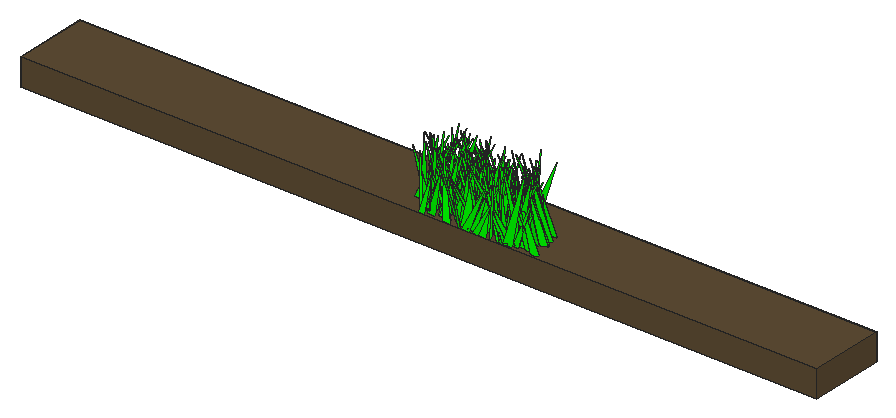
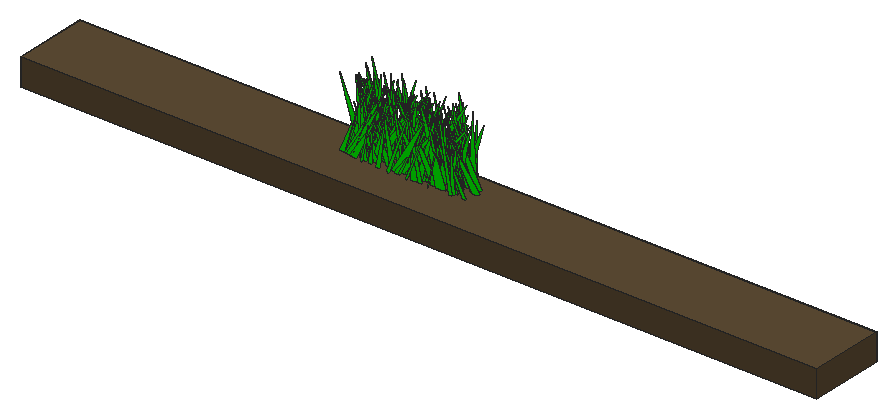
# SketchUp Ruby script. Lengths in inches.
U = 1.inch
M = Sketchup.active_model
def pt(a) = Geom::Point3d.new(a.map { |v| v * U })
def face(e, loops, mat)
  f = e.add_face(loops[0].map { |a| pt(a) })
  loops[1..].each { |l| e.add_face(l.map { |a| pt(a) }).erase! }
  f.material = f.back_material = mat if mat
  f
end
# faces: each face lists its corners as indices into pts; further lists are holes
def faces(e, pts, list, mat = nil) = list.each { |f| face(e, (f[0].is_a?(Array) ? f : [f]).map { |l| l.map { |i| pts[i] } }, mat) }
# xy, xz, yz: faces in a plane at the given z, y or x. An outline is a flat list of corners, or four numbers for a rectangle; further outlines are holes
def ring(l) = l.size == 4 ? [[l[0], l[1]], [l[2], l[1]], [l[2], l[3]], [l[0], l[3]]] : l.each_slice(2).to_a
def flat(e, list, mat, &to3) = list.each { |f| face(e, (f[0].is_a?(Array) ? f : [f]).map { |l| ring(l).map { |u, v| to3.(u, v) } }, mat) }
def xy(e, z, list, mat = nil) = flat(e, list, mat) { |x, y| [x, y, z] }
def xz(e, y, list, mat = nil) = flat(e, list, mat) { |x, z| [x, y, z] }
def yz(e, x, list, mat = nil) = flat(e, list, mat) { |y, z| [x, y, z] }
def lines(e, pts, list) = list.each { |a, b| e.add_line(pt(pts[a]), pt(pts[b])) }
# prism: a flat outline (further loops are holes) pulled along v
def prism(e, loops, v, mat = nil)
  f = face(e, loops, mat); d = Geom::Vector3d.new(v.map { |x| x * U })
  f.pushpull(f.normal.samedirection?(d) ? d.length : -d.length)
end
def box(e, o, s, mat = nil) = prism(e, [[o, [o[0] + s[0], o[1], o[2]], [o[0] + s[0], o[1] + s[1], o[2]], [o[0], o[1] + s[1], o[2]]]], [0, 0, s[2]], mat)
def at(x, y, z, deg = 0) = Geom::Transformation.translation(pt([x, y, z])) * Geom::Transformation.rotation(ORIGIN, Z_AXIS, deg.degrees)
def axes(o, x, y, z) = Geom::Transformation.new([*x, 0, *y, 0, *z, 0, *pt(o).to_a, 1])
def part(name) = M.definitions.add(name)
# library, detail: a bought-in or finely detailed component or shape, given as its bounding box
def library(name, o, s) = part(name).tap { |d| box(d.entities, o, s) }
def detail(e, o, s) = box(e.add_group.entities, o, s)
def put(e, d, t, mat = nil) = e.add_instance(d, t).tap { |i| i.material = mat if mat }
def group(e, t, mat = nil) = e.add_group.tap { |g| g.transformation = t; g.material = mat if mat }.entities
root = M.entities
M.materials.add("SOIL").color = [94, 77, 53]
M.materials.add("[0065_Lime]").color = [0, 255, 0]
c1 = part("fur_instance\#9")
p = [[0.8125,0,1.79],[0.67,-0.02,1.48],[0,-0.11,0],[0,0.11,0]]
faces(c1.entities,p,[[0,1,2,3]])
c2 = part("SOIL")
box(c2.entities,[0,0,0],[23.62,15.75,0.98],"SOIL")
put(root,c1,axes([86.26,21.52,1.48],[-3.92329,-0.98514,1.62237],[6.99474,-0.59837,-0.98359],[2.05017,0.15629,6.46044]),"[0065_Lime]")
put(root,c1,axes([87.06,25.03,1.48],[-4.86713,-0.43514,0.69437],[2.59385,-0.66086,-1.84784],[1.89478,-0.21307,4.31322]),"[0065_Lime]")
put(root,c1,axes([86.95,25.65,1.48],[-3.6434,0.55108,0.79164],[-3.69089,-0.52882,1.0962],[1.64458,0.03404,4.21395]),"[0065_Lime]")
put(root,c1,axes([88.84,19.94,1.48],[-2.13594,0.89801,1.23841],[-6.47476,-0.24967,-1.32207],[-1.11202,-0.27113,5.3191]),"[0065_Lime]")
put(root,c1,axes([87.3,25.59,1.48],[3.80102,-0.6268,0.11207],[4.06406,0.49666,1.88228],[-1.84392,-0.19742,4.37965]),"[0065_Lime]")
put(root,c1,axes([88.48,23.02,1.48],[2.15335,-0.98377,0.49833],[6.63438,0.31426,1.82077],[-2.31848,-0.01445,5.67301]),"[0065_Lime]")
put(root,c1,axes([84.02,23.47,1.48],[2.87828,0.89252,1.10575],[-6.05727,0.29337,2.49735],[2.34533,-0.33764,5.09286]),"[0065_Lime]")
put(root,c1,axes([87.92,18.82,1.48],[-6.21024,0.38109,1.41418],[-2.17849,-0.88765,1.68567],[2.37317,0.18242,5.24809]),"[0065_Lime]")
put(root,c1,axes([84.51,22.2,1.48],[7.67509,-0.55885,1.19656],[4.23893,1.02256,-1.98637],[-0.11322,0.40028,6.745]),"[0065_Lime]")
put(root,c1,axes([89.35,23.6,1.48],[-1.78988,0.89977,2.25183],[-6.87567,-0.15965,-1.4784],[-1.17922,-0.43485,5.20214]),"[0065_Lime]")
put(root,c1,axes([87.04,24.39,1.48],[-4.0744,0.73037,0.72448],[-4.66339,-0.57286,1.9996],[2.46223,0.12362,4.98603]),"[0065_Lime]")
put(root,c2,axes([7.75,33.48,-3.9375],[6.76163,0,0],[0,-0.95013,0],[0,0,5.5]),"[0065_Lime]")
put(root,c1,axes([84.83,23.29,1.48],[6.25065,0.54898,1.04221],[-4.0981,0.80537,2.0467],[0.33236,-0.39401,5.63564]),"[0065_Lime]")
put(root,c1,axes([87.84,22.97,1.48],[4.78661,-0.31487,1.61147],[1.83054,0.72385,1.14181],[-2.3654,-0.07699,4.1446]),"[0065_Lime]")
put(root,c1,axes([88.79,23.93,1.48],[2.13807,-0.60622,1.20283],[4.12647,0.35487,1.14015],[-1.942,0.08662,3.74691]),"[0065_Lime]")
put(root,c1,axes([84.52,25.74,1.48],[8.40774,0.5005,0.59305],[-3.63094,1.14274,1.74246],[0.18567,-0.3169,7.22006]),"[0065_Lime]")
put(root,c1,axes([87.15,26.11,1.48],[8.38516,-0.29232,1.59438],[1.78727,1.20242,1.16821],[-2.23058,-0.13545,6.9296]),"[0065_Lime]")
put(root,c1,axes([86.33,22.54,1.48],[2.78842,-0.77084,0.42707],[5.3628,0.36053,-1.3615],[1.26859,0.17025,4.81682]),"[0065_Lime]")
put(root,c1,axes([86.59,21.64,1.48],[4.73426,-0.22221,0.40328],[1.65265,0.61725,-1.43981],[0.12388,0.25771,3.79619]),"[0065_Lime]")
put(root,c1,axes([88.5,20.06,1.48],[-3.34713,1.10893,1.52084],[-7.9031,-0.5098,0.94778],[1.82118,-0.17419,6.90805]),"[0065_Lime]")
put(root,c1,axes([90,23.15,1.48],[-7.34801,-0.13765,1.45115],[0.23204,-0.98967,-2.36838],[2.02201,-0.38666,5.54526]),"[0065_Lime]")
put(root,c1,axes([86.69,25.4375,1.48],[4.16394,-0.68264,0.5679],[4.88041,0.56231,-1.02707],[0.51896,0.18917,5.10214]),"[0065_Lime]")
put(root,c1,axes([88.16,23.67,1.48],[5.57945,0.19788,1.87781],[-2.1365,0.77852,1.45115],[-1.65766,-0.33737,4.45009]),"[0065_Lime]")
put(root,c1,axes([88.4,20.36,1.48],[7.19257,-0.02911,2.1896],[-0.66477,1.02413,1.90098],[-2.6167,-0.34018,5.53564]),"[0065_Lime]")
put(root,c1,axes([87.36,20.45,1.48],[-0.41032,-1.05692,2.34051],[7.77509,-0.15747,-1.48095],[2.09816,0.37684,5.94562]),"[0065_Lime]")
put(root,c1,axes([88.17,18.53,1.48],[-1.51213,0.71533,0.74035],[-4.88132,-0.24143,1.22024],[1.70763,-0.05671,4.1437]),"[0065_Lime]")
put(root,c1,axes([88.54,21.08,1.48],[-4.71965,1.1231,1.02402],[-7.5613,-0.68511,2.12056],[2.87973,0.04178,7.24622]),"[0065_Lime]")
put(root,c1,axes([90.3,24.2,1.48],[-6.08915,-0.43152,0.27868],[2.58805,-0.77035,-2.55579],[1.68816,-0.37548,4.92338]),"[0065_Lime]")
put(root,c1,axes([90.07,24.21,1.48],[-7.13212,0.8292,0.16302],[-5.37474,-0.93003,2.93686],[2.44437,0.37445,6.9333]),"[0065_Lime]")
put(root,c1,axes([86.86,22.75,1.48],[8.90731,-0.03099,1.00216],[-0.24418,1.17722,2.65579],[-1.22758,-0.45903,6.74342]),"[0065_Lime]")
put(root,c1,axes([88.23,19.93,1.48],[-1.89386,-1.1692,2.55973],[8.62726,-0.35166,-1.15923],[2.16966,0.37774,6.84378]),"[0065_Lime]")
put(root,c1,axes([91.72,21.7,1.48],[-3.06722,0.66122,1.4293],[-4.94736,-0.34767,-1.63498],[-0.86839,-0.35475,4.26639]),"[0065_Lime]")
put(root,c1,axes([94.47,23.15,1.48],[-5.84379,-0.90349,0.13146],[5.9457,-0.74716,2.80522],[-2.45278,0.34142,6.48682]),"[0065_Lime]")
put(root,c1,axes([92.15,21.19,1.48],[-7.16805,0.35651,1.21602],[-2.84625,-0.98057,-1.46757],[0.75551,-0.31166,6.00841]),"[0065_Lime]")
put(root,c1,axes([86.89,23.54,1.48],[4.54611,0.66185,0.06214],[-4.50822,0.60694,1.60163],[1.36625,-0.19953,5.07813]),"[0065_Lime]")
put(root,c1,axes([88.17,18.84,1.48],[5.37977,0.10536,0.4433],[-0.85123,0.74006,0.94123],[-0.36685,-0.17218,4.31685]),"[0065_Lime]")
put(root,c1,axes([89.24,21.59,1.48],[6.91772,0.2578,1.35724],[-1.3471,0.97398,-1.65641],[-2.08217,0.22638,5.58087]),"[0065_Lime]")
put(root,c1,axes([89.15,23.03,1.48],[5.45261,-0.71154,2.28127],[5.66523,0.76712,-0.94152],[-1.18829,0.39228,5.97914]),"[0065_Lime]")
put(root,c1,axes([88.37,23.62,1.48],[5.83953,-0.0187,0.3522],[0.25645,0.78495,-1.41702],[-0.37339,0.24672,4.53495]),"[0065_Lime]")
put(root,c1,axes([87.99,22.96,1.48],[1.38405,1.28333,0.05786],[-8.80843,0.18489,1.99424],[2.41381,-0.06115,7.24416]),"[0065_Lime]")
put(root,c1,axes([91.53,26.2,1.48],[-5.38065,-0.09729,1.13702],[0.30877,-0.75789,-1.20625],[1.52904,-0.18931,4.24471]),"[0065_Lime]")
put(root,c1,axes([89.6,19.23,1.48],[-0.92109,-0.87068,0.19494],[5.93364,-0.13365,-1.45203],[1.80077,-0.00498,4.88422]),"[0065_Lime]")
put(root,c1,axes([89.98,24.79,1.48],[6.48922,0.77798,0.48487],[-5.27514,0.90004,-1.67983],[-1.78365,0.16855,6.73211]),"[0065_Lime]")
put(root,c1,axes([93.01,19.42,1.48],[-5.11478,0.39,0.82683],[-2.95192,-0.68846,-1.20065],[0.14956,-0.25096,4.57867]),"[0065_Lime]")
put(root,c1,axes([87.44,23.39,1.48],[5.95821,-0.99713,0.91696],[7.05524,0.77298,-2.16565],[1.3597,0.35854,7.21907]),"[0065_Lime]")
put(root,c1,axes([91.85,23.32,1.48],[-4.79332,0.08655,1.09953],[-0.29385,-0.68424,0.95724],[1.45611,0.14683,3.81268]),"[0065_Lime]")
put(root,c1,axes([88.75,22.9,1.48],[3.65247,0.5864,0.04969],[-3.99548,0.48798,1.34531],[1.20623,-0.15924,4.30573]),"[0065_Lime]")
put(root,c1,axes([92.36,25.01,1.48],[1.24089,-0.74454,0.2399],[5.06099,0.17884,1.27788],[-1.59625,-0.01178,4.23806]),"[0065_Lime]")
put(root,c1,axes([95.9,21.22,1.48],[-4.24202,-1.17622,0.85066],[8.0481,-0.51501,2.69181],[-2.52777,0.33416,7.14283]),"[0065_Lime]")
put(root,c1,axes([89.41,25.5625,1.48],[1.69744,-1.29614,0.1512],[9.00225,0.22688,-1.69681],[2.01919,0.07811,7.43786]),"[0065_Lime]")
put(root,c1,axes([91.96,24.03,1.48],[-2.77196,-0.41389,0.48866],[2.7405,-0.39512,-0.92866],[1.23551,-0.05218,3.15624]),"[0065_Lime]")
put(root,c1,axes([90.42,22.3125,1.48],[6.60326,0.23677,1.73332],[-2.39513,0.87879,2.01468],[-1.28193,-0.42231,5.16422]),"[0065_Lime]")
put(root,c1,axes([90.89,19.94,1.48],[6.17113,-0.37454,0.65547],[2.29185,0.83954,1.79843],[-1.58158,-0.24485,5.16367]),"[0065_Lime]")
put(root,c1,axes([93.65,23.65,1.48],[-5.17463,-0.20057,1.12461],[1.83055,-0.69199,1.43748],[0.77326,0.29598,4.12289]),"[0065_Lime]")
put(root,c1,axes([93.02,18.65,1.48],[-6.14592,0.83652,0.11307],[-5.59721,-0.82111,2.26538],[2.03236,0.26828,6.5809]),"[0065_Lime]")
put(root,c1,axes([94.13,25.13,1.48],[-5.65127,-0.76849,1.90898],[5.91576,-0.77501,1.13269],[0.64923,0.37245,6.29582]),"[0065_Lime]")
put(root,c1,axes([94.52,19.5625,1.48],[-7.703,-0.60503,0.28827],[4.04129,-1.04509,-2.05032],[1.52732,-0.28614,6.87907]),"[0065_Lime]")
put(root,c1,axes([90.77,22.96,1.48],[3.19064,-0.8803,1.7455],[6.57368,0.38069,-1.51707],[0.79863,0.38342,5.51372]),"[0065_Lime]")
put(root,c1,axes([91.61,20.05,1.48],[-0.87029,0.95899,1.84974],[-6.97198,-0.19173,1.16039],[1.77181,-0.28338,5.47463]),"[0065_Lime]")
put(root,c1,axes([89.73,22.98,1.48],[8.53271,-0.01095,0.23182],[0.13342,1.1753,-1.38965],[-0.26361,0.24054,6.80037]),"[0065_Lime]")
put(root,c1,axes([91.88,19.71,1.48],[-0.80568,1.10588,0.25369],[-7.66296,-0.12024,1.462],[1.82035,-0.01672,6.26676]),"[0065_Lime]")
put(root,c1,axes([91.4,20.93,1.48],[-2.08798,-1.19343,1.13044],[8.01876,-0.34275,-2.32557],[3.12474,0.08211,6.72328]),"[0065_Lime]")
put(root,c1,axes([93.16,25.02,1.48],[4.07601,-0.64978,0.15995],[4.34934,0.55033,1.58152],[-1.5827,-0.16108,4.75806]),"[0065_Lime]")
put(root,c1,axes([94.65,22.58,1.48],[0.1089,0.80647,0.27548],[-5.57394,0.02647,-1.1392],[-1.40894,-0.0424,4.52813]),"[0065_Lime]")
put(root,c1,axes([93.375,21.8125,1.48],[7.43188,0.70493,1.48792],[-4.33925,1.05401,-2.39275],[-3.11192,0.21381,6.88989]),"[0065_Lime]")
put(root,c1,axes([91.58,22.57,1.48],[1.24779,-0.82828,0.7168],[5.70231,0.12912,-1.56833],[1.73345,0.17148,4.64317]),"[0065_Lime]")
put(root,c1,axes([91.73,23.09,1.48],[0.08522,-1.01564,0.05164],[6.91268,0.00885,-1.71857],[2.11201,0.01203,5.62286]),"[0065_Lime]")
put(root,c1,axes([97.71,25.11,1.48],[-6.24236,-0.70374,0.25657],[4.78633,-0.81375,2.25756],[-1.50739,0.33045,6.1058]),"[0065_Lime]")
put(root,c1,axes([95.73,24.32,1.48],[-3.1177,-1.13474,1.55341],[8.28426,-0.40903,0.98862],[-0.48009,0.31085,6.97144]),"[0065_Lime]")
put(root,c1,axes([90.82,25.25,1.48],[7.23919,-0.64046,0.74671],[4.62979,0.97112,-1.78689],[0.42637,0.32915,6.72501]),"[0065_Lime]")
put(root,c1,axes([95.73,26.38,1.48],[-5.65432,-0.04845,0.63646],[0.10921,-0.77024,-1.32264],[0.84804,-0.22382,4.41394]),"[0065_Lime]")
put(root,c1,axes([96.75,21.36,1.48],[-8.8985,0.03558,1.49879],[-0.89066,-1.19251,-2.55005],[1.63278,-0.45657,6.77721]),"[0065_Lime]")
put(root,c1,axes([93.27,26.12,1.48],[7.23996,0.4968,2.08933],[-4.02026,1.03099,1.00264],[-1.71321,-0.31987,6.47661]),"[0065_Lime]")
put(root,c1,axes([96.125,25.16,1.48],[-5.21387,-0.42168,1.80804],[3.65708,-0.68514,1.62321],[0.75617,0.40607,4.61626]),"[0065_Lime]")
put(root,c1,axes([94.39,26.11,1.48],[-1.25887,-0.73596,0.02909],[5.12309,-0.1741,-0.90453],[1.08943,-0.03174,4.28722]),"[0065_Lime]")
put(root,c1,axes([97.52,22.12,1.48],[-6.30277,0.84398,0.95995],[-6.1205,-0.86568,-1.0847],[-0.0841,-0.24995,6.99826]),"[0065_Lime]")
put(root,c1,axes([94.93,23.12,1.48],[4.53966,0.16692,1.46941],[-0.78928,0.67756,-0.96577],[-2.01283,0.11078,3.69275]),"[0065_Lime]")
put(root,c1,axes([95.58,18.63,1.48],[-4.56773,-0.28709,0.83866],[1.72242,-0.64423,-1.18296],[1.50683,-0.13386,3.89449]),"[0065_Lime]")
put(root,c1,axes([98.3,25.84,1.48],[-1.04289,1.11947,0.73824],[-7.45065,-0.08777,-2.50423],[-2.96322,-0.17331,6.03674]),"[0065_Lime]")
put(root,c1,axes([98.41,25.9,1.48],[-6.03014,-0.55616,0.99177],[4.09114,-0.75289,2.31058],[-0.64386,0.42484,5.39306]),"[0065_Lime]")
put(root,c1,axes([94.375,25.27,1.48],[7.41064,-0.405,0.78932],[2.25405,0.97257,2.71982],[-2.04154,-0.3963,5.8681]),"[0065_Lime]")
put(root,c1,axes([93.5,21.03,1.48],[0.87194,-1.14502,0.68618],[7.96685,0.09075,-1.62352],[1.90804,0.14431,6.46529]),"[0065_Lime]")
put(root,c1,axes([97.49,24.32,1.48],[-1.17805,0.9444,0.81244],[-6.65002,-0.13102,-1.27663],[-1.39456,-0.17302,5.40136]),"[0065_Lime]")
put(root,c1,axes([99.01,19.73,1.48],[-0.87813,-0.84769,1.0208],[5.33727,-0.01563,2.60285],[-3.07907,0.21466,4.22065]),"[0065_Lime]")
put(root,c1,axes([94.71,20.59,1.48],[7.676,-0.64027,0.89714],[4.17245,1.0686,1.93467],[-2.13744,-0.21333,6.99845]),"[0065_Lime]")
put(root,c1,axes([97.07,21.32,1.48],[-6.08511,-0.47059,0.39218],[2.92815,-0.80228,-2.1984],[1.69537,-0.30342,5.20457]),"[0065_Lime]")
put(root,c1,axes([98.37,23.99,1.48],[-5.66498,-0.36701,0.7544],[2.76604,-0.76747,1.2316],[0.17613,0.24827,4.92241]),"[0065_Lime]")
put(root,c1,axes([97.88,24.25,1.48],[-2.3622,-0.88866,1.1995],[6.46398,-0.30066,0.95852],[-0.62186,0.25044,5.40699]),"[0065_Lime]")
put(root,c1,axes([97.61,24.2,1.48],[2.34346,1.00533,2.89602],[-7.63303,0.43597,-0.98458],[-2.36628,-0.41068,6.04411]),"[0065_Lime]")
put(root,c1,axes([93.29,25.06,1.48],[5.0037,-0.85593,0.94511],[6.02233,0.62074,-2.25822],[1.47814,0.36837,6.00125]),"[0065_Lime]")
put(root,c1,axes([96.97,25.04,1.48],[-7.6324,-0.46133,2.07648],[2.73169,-1.12143,-1.70536],[3.13582,-0.14596,6.5396]),"[0065_Lime]")
put(root,c1,axes([99.21,21.3,1.48],[-1.87029,-0.57707,0.06333],[3.68905,-0.23071,1.63992],[-1.80619,0.12634,3.28388]),"[0065_Lime]")
put(root,c1,axes([96.39,19.21,1.48],[-2.77506,1.0906,0.7454],[-7.52252,-0.4098,1.56158],[2.11889,-0.02653,6.52019]),"[0065_Lime]")
put(root,c1,axes([97.75,21.77,1.48],[4.00428,-0.77201,0.3209],[4.98082,0.53676,2.14824],[-2.352,-0.17767,5.09564]),"[0065_Lime]")
put(root,c1,axes([99.36,26.46,1.48],[-7.84255,0.10057,1.34447],[-1.16401,-1.07481,-1.7985],[1.37451,-0.33641,6.14808]),"[0065_Lime]")
put(root,c1,axes([96.43,22.79,1.48],[1.57206,-0.7285,0.73516],[5.17743,0.19034,-1.00476],[0.94307,0.1694,4.29062]),"[0065_Lime]")
put(root,c1,axes([98.5,24.09,1.48],[-8.09034,-0.04073,2.66504],[-1.23983,-1.09449,-3.05076],[3.04654,-0.55357,5.83569]),"[0065_Lime]")
put(root,c1,axes([97.82,20.32,1.48],[-5.02165,1.01793,0.04543],[-6.82181,-0.66767,2.38317],[2.43794,0.22847,6.76212]),"[0065_Lime]")
put(root,c1,axes([99.39,19.26,1.48],[-4.09321,-0.73209,1.66853],[5.59019,-0.55457,0.92003],[0.3176,0.32611,5.31019]),"[0065_Lime]")
put(root,c1,axes([98.09,24.37,1.48],[4.50376,0.16636,1.43326],[-0.56089,0.65334,-1.37497],[-2.04738,0.18696,3.52951]),"[0065_Lime]")
put(root,c1,axes([97.34,18.69,1.48],[4.22997,0.0853,0.47642],[-0.26358,0.53342,-1.65194],[-0.8013,0.27483,3.05834]),"[0065_Lime]")
put(root,c1,axes([95.43,21.96,1.48],[1.97167,1.15444,0.80354],[-7.92004,0.22194,2.17327],[2.39702,-0.21626,6.5198]),"[0065_Lime]")
put(root,c1,axes([97.8,24.31,1.48],[6.35269,0.73648,0.3431],[-4.79464,0.84952,-2.36675],[-2.1585,0.2805,6.267]),"[0065_Lime]")
put(root,c1,axes([98.86,21.97,1.48],[-6.83338,-0.30879,1.70341],[1.37367,-0.96094,-2.19114],[2.70695,-0.29187,5.41197]),"[0065_Lime]")
put(root,c1,axes([97.33,19.5,1.48],[-0.51866,-0.58562,1.68295],[4.36727,-0.16219,-1.00063],[1.60515,0.25205,3.26629]),"[0065_Lime]")
put(root,c1,axes([98.12,20.77,1.48],[-2.27643,-0.86264,0.24382],[5.94097,-0.32034,-1.27762],[1.57542,-0.03848,5.17028]),"[0065_Lime]")
put(root,c1,axes([98.64,21.64,1.48],[5.96405,0.5779,1.60011],[-3.6968,0.87941,-1.52603],[-2.6678,0.07332,5.6918]),"[0065_Lime]")
put(root,c1,axes([100.92,20.62,1.48],[-4.7806,0.17181,0.19589],[-1.24523,-0.65337,-0.90453],[-0.04855,-0.15973,3.91052]),"[0065_Lime]")
put(root,c1,axes([96.98,18.53,1.48],[2.19958,-0.8129,0.37175],[5.63211,0.2825,-1.34922],[1.39817,0.14089,4.85011]),"[0065_Lime]")
put(root,c1,axes([99.8,20.91,1.48],[-7.38587,-0.12209,2.68193],[2.026,-1.04621,2.09574],[2.74249,0.44409,5.67455]),"[0065_Lime]")
put(root,c1,axes([96.08,20.95,1.48],[3.35159,-0.87386,0.08675],[5.84909,0.43703,-1.99809],[2.11519,0.17615,5.38782]),"[0065_Lime]")
put(root,c1,axes([103.55,20.99,1.48],[-5.95619,0.95247,0.06297],[-6.49172,-0.79729,-2.16609],[-1.95164,-0.25482,7.01284]),"[0065_Lime]")
put(root,c1,axes([103.34,24.05,1.48],[-3.09142,1.1109,0.87784],[-7.41255,-0.33966,-2.8683],[-2.95303,-0.31037,6.28089]),"[0065_Lime]")
put(root,c1,axes([102,24.24,1.48],[-1.85161,0.48227,0.9328],[-3.15808,-0.12699,-1.94756],[-1.76664,-0.27845,2.50382]),"[0065_Lime]")
put(root,c1,axes([99.42,25.36,1.48],[-4.25525,0.66632,0.9482],[-4.2179,-0.61103,1.86413],[2.46042,0.1049,4.83557]),"[0065_Lime]")
put(root,c1,axes([102.96,22.83,1.48],[-1.21971,-1.20922,1.12379],[8.2502,-0.09698,2.42782],[-2.81021,0.24012,6.63983]),"[0065_Lime]")
put(root,c1,axes([98.99,23.98,1.48],[8.17537,-0.5417,1.77311],[3.57711,1.18685,1.23748],[-2.61096,-0.07012,7.2473]),"[0065_Lime]")
put(root,c1,axes([98.2,18.93,1.48],[4.61367,0.56143,1.35377],[-4.32738,0.60508,1.34919],[-0.08527,-0.32996,4.7776]),"[0065_Lime]")
put(root,c1,axes([97.39,19.27,1.48],[2.71581,0.79689,0.80285],[-5.43594,0.30459,2.03571],[1.89376,-0.26851,4.69204]),"[0065_Lime]")
put(root,c1,axes([101.67,24.22,1.48],[-5.67209,-0.41872,0.31145],[2.83432,-0.78391,-1.16261],[0.99635,-0.15372,5.08036]),"[0065_Lime]")
put(root,c1,axes([98.8,20.22,1.48],[-2.53944,1.15947,1.24248],[-7.85549,-0.40733,2.11429],[2.95133,-0.08652,6.69663]),"[0065_Lime]")
put(root,c1,axes([98.64,23.79,1.48],[0.04142,-1.24747,0.27902],[8.64107,-0.00555,-1.67954],[2.06476,0.04823,7.02329]),"[0065_Lime]")
put(root,c1,axes([98.94,18.53,1.48],[1.64861,-0.61939,0.01021],[4.25007,0.22286,-1.01894],[1.16906,0.06325,3.68992]),"[0065_Lime]")
put(root,c1,axes([100.73,20.8125,1.48],[-6.33679,-0.12856,2.64813],[1.85552,-0.9445,1.40129],[2.82716,0.33174,5.01581]),"[0065_Lime]")
put(root,c1,axes([99.32,25.1,1.48],[7.33111,0.5697,0.58756],[-3.71258,1.00399,-1.97087],[-1.78205,0.25203,6.52312]),"[0065_Lime]")
put(root,c1,axes([99.875,20.45,1.48],[-7.05777,0.3073,4.2308],[-3.66226,-1.1399,-1.26777],[4.29232,-0.46728,5.87494]),"[0065_Lime]")
put(root,c1,axes([101.4375,26.37,1.48],[-4.55952,-0.52207,0.25388],[3.36525,-0.60608,-1.77492],[1.60501,-0.2123,4.44271]),"[0065_Lime]")
put(root,c1,axes([102.86,24.08,1.48],[-1.26384,-0.668,1.69382],[5.00362,-0.07687,1.45437],[-1.37799,0.33354,3.72746]),"[0065_Lime]")
put(root,c1,axes([100.18,18.63,1.48],[-3.29917,0.96248,1.81688],[-6.73721,-0.53447,1.39307],[2.55256,-0.16666,6.02518]),"[0065_Lime]")
put(root,c1,axes([102.88,25.11,1.48],[-0.30218,1.02501,0.01193],[-7.08174,-0.04073,-1.42447],[-1.74914,-0.01218,5.76519]),"[0065_Lime]")
put(root,c1,axes([98.86,21.72,1.48],[1.56936,0.77965,0.13485],[-5.15439,0.19569,1.77621],[2.06033,-0.10429,4.3409]),"[0065_Lime]")
put(root,c1,axes([102.6,23.88,1.48],[-0.46541,-0.67925,0.80479],[4.79322,-0.0291,1.0109],[-1.17082,0.15086,3.81862]),"[0065_Lime]")
put(root,c1,axes([105.82,19.08,1.48],[-3.83955,-1.08206,1.19782],[7.15016,-0.38878,3.3958],[-3.21583,0.4275,6.12016]),"[0065_Lime]")
put(root,c1,axes([100.08,24.42,1.48],[6.78058,-0.36528,0.89028],[2.38146,0.95599,1.1431],[-1.5114,-0.13245,5.79519]),"[0065_Lime]")
put(root,c1,axes([104.03,20.51,1.48],[-0.36574,0.91391,0.04257],[-5.99315,-0.04449,-2.06085],[-2.52696,-0.02675,4.88152]),"[0065_Lime]")
put(root,c1,axes([103.39,18.97,1.48],[-7.73295,0.30324,1.63976],[-2.49915,-1.095,-1.01235],[1.5733,-0.2489,6.45149]),"[0065_Lime]")
put(root,c1,axes([105.0625,25.14,1.48],[-8.00811,0.148,0.22883],[-1.08996,-1.08086,-1.81227],[-0.02261,-0.31554,6.31511]),"[0065_Lime]")
put(root,c1,axes([101.41,22.51,1.48],[5.03268,-0.56586,0.1756],[3.60552,0.65309,2.15048],[-1.8064,-0.27295,4.7815]),"[0065_Lime]")
put(root,c1,axes([98.78,20.85,1.48],[7.35861,0.0694,0.00183],[-0.48668,1.01806,1.04958],[0.0842,-0.18093,5.90653]),"[0065_Lime]")
put(root,c1,axes([100.16,25.01,1.48],[1.67556,0.86074,0.15574],[-5.98872,0.22404,1.13842],[1.3013,-0.07723,5.03858]),"[0065_Lime]")
put(root,c1,axes([99.48,22.28,1.48],[4.68078,0.4722,0.42514],[-3.30948,0.60369,1.64014],[0.78303,-0.27123,4.39066]),"[0065_Lime]")
put(root,c1,axes([101.66,19.1,1.48],[6.60094,-0.29038,1.39974],[1.16814,0.88691,2.52049],[-2.42219,-0.36361,5.03009]),"[0065_Lime]")
put(root,c1,axes([102.95,19.47,1.48],[-5.63328,0.50589,1.01603],[-3.40954,-0.80902,0.99052],[1.70201,0.05374,5.34707]),"[0065_Lime]")
put(root,c1,axes([103.88,18.81,1.48],[-4.61026,-0.28166,0.95397],[2.28192,-0.61745,1.1878],[0.4313,0.25611,3.91283]),"[0065_Lime]")
put(root,c1,axes([104.55,24.85,1.48],[-8.59378,0.11297,1.18282],[-0.17605,-1.13223,2.77744],[1.65226,0.46697,6.44808]),"[0065_Lime]")
put(root,c1,axes([104.52,18.87,1.48],[0.6572,-0.58632,1.75788],[4.06906,0.22437,1.50119],[-2.35027,0.22451,3.09059]),"[0065_Lime]")
put(root,c1,axes([102.83,20.47,1.48],[7.68548,-0.18643,2.64573],[-0.03617,1.0952,2.65553],[-3.51263,-0.41918,5.7614]),"[0065_Lime]")
put(root,c1,axes([104.34,23.21,1.48],[-5.33073,-0.15477,0.40759],[0.97109,-0.73695,-0.97365],[0.72193,-0.15152,4.31929]),"[0065_Lime]")
put(root,c1,axes([102.05,21.53,1.48],[-2.08888,-1.28209,0.35299],[8.95404,-0.29977,-1.42624],[1.80615,0.00335,7.47887]),"[0065_Lime]")
put(root,c1,axes([102.09,20.38,1.48],[-2.8781,1.14966,1.67959],[-8.01358,-0.46842,1.65836],[2.643,-0.16831,6.85713]),"[0065_Lime]")
put(root,c1,axes([103.25,26.0625,1.48],[3.21349,-0.43408,0.14923],[2.75621,0.41837,1.50898],[-1.40698,-0.17184,3.29685]),"[0065_Lime]")
put(root,c1,axes([102.66,23.24,1.48],[3.77028,0.37382,0.04015],[-2.47451,0.49704,-1.3265],[-0.97798,0.18351,3.51115]),"[0065_Lime]")
put(root,c1,axes([105.3,23.43,1.48],[-1.22014,-0.89532,1.59504],[6.55536,-0.1102,1.2451],[-1.21218,0.30525,5.1279]),"[0065_Lime]")
put(root,c1,axes([105.32,24.91,1.48],[-1.06531,-0.75887,0.37633],[5.26561,-0.12918,1.13372],[-1.28563,0.09974,4.33159]),"[0065_Lime]")
put(root,c1,axes([103.77,19.91,1.48],[3.4079,-0.67512,0.2912],[4.55233,0.4714,1.37255],[-1.57729,-0.09812,4.59055]),"[0065_Lime]")
put(root,c1,axes([103.63,20.43,1.48],[-3.3739,0.39943,0.71085],[-2.37754,-0.47385,1.45572],[1.78638,0.12374,3.28003]),"[0065_Lime]")
put(root,c1,axes([104.67,26.48,1.48],[-5.7971,-0.13922,1.31156],[0.18444,-0.76817,-2.19299],[1.88349,-0.35328,4.25155]),"[0065_Lime]")
put(root,c1,axes([105.83,25.53,1.48],[-5.33549,-0.18278,0.07603],[1.24258,-0.72932,-1.05607],[0.39579,-0.17425,4.34044]),"[0065_Lime]")
put(root,c1,axes([105.41,22.69,1.48],[-7.20546,-0.38101,0.99441],[2.40461,-1.0112,-1.45452],[1.75057,-0.17927,6.091]),"[0065_Lime]")
put(root,c1,axes([104.44,22.74,1.48],[4.18283,-0.08146,1.6329],[-0.11254,0.62152,1.22971],[-2.08647,-0.19683,3.20722]),"[0065_Lime]")
put(root,c1,axes([106.7,26.08,1.48],[-2.50151,0.68862,0.74053],[-4.77412,-0.28987,-1.63792],[-1.43269,-0.23643,4.16502]),"[0065_Lime]")
put(root,c1,axes([107.36,25.9,1.48],[-3.78597,0.85892,0.49517],[-5.95826,-0.48903,-1.71676],[-1.49427,-0.22624,5.59083]),"[0065_Lime]")
put(root,c1,axes([102.53,25.32,1.48],[7.99103,-0.52341,0.69339],[3.54015,1.1186,1.30014],[-1.43826,-0.15475,7.05264]),"[0065_Lime]")
put(root,c1,axes([104.87,23.94,1.48],[-3.97558,-0.44726,0.61367],[2.9163,-0.56019,-1.18094],[1.48179,-0.09749,3.97065]),"[0065_Lime]")
put(root,c1,axes([107.82,25.74,1.48],[-5.47396,0.83992,1.29888],[-6.09837,-0.68198,-2.22728],[-1.04312,-0.4206,6.20517]),"[0065_Lime]")
put(root,c1,axes([105.6,23.02,1.48],[-6.6588,-0.7284,0.42861],[4.81464,-0.90611,-2.10955],[1.99188,-0.24484,6.53188]),"[0065_Lime]")
put(root,c1,axes([107.28,25.0625,1.48],[-8.82172,0.15589,0.72013],[-0.6671,-1.14665,2.91054],[1.2528,0.48713,6.6207]),"[0065_Lime]")
put(root,c1,axes([105.61,22.5,1.48],[2.7481,-0.69445,0.80221],[4.61266,0.41019,1.44393],[-2.02991,-0.00806,4.36716]),"[0065_Lime]")
put(root,c1,axes([102.57,25.21,1.48],[3.68509,-0.70012,0.89219],[5.01017,0.46077,-1.57599],[0.96241,0.28211,4.78816]),"[0065_Lime]")
put(root,c1,axes([107.24,19.85,1.48],[-1.50021,1.17889,0.52111],[-8.23755,-0.18715,-1.50328],[-1.71431,-0.13235,6.76751]),"[0065_Lime]")
put(root,c1,axes([104.68,25.76,1.48],[6.38928,-0.67686,1.56561],[4.66727,0.93739,0.97745],[-2.26351,0.02229,6.43477]),"[0065_Lime]")
put(root,c1,axes([109.53,22.56,1.48],[-3.18639,0.95668,0.7066],[-6.16445,-0.33974,-2.97919],[-3.01776,-0.31615,5.33957]),"[0065_Lime]")
put(root,c1,axes([105.23,25.29,1.48],[-7.18362,0.69109,2.81224],[-4.57467,-1.11953,1.48721],[3.90053,-0.04023,6.92358]),"[0065_Lime]")
put(root,c1,axes([104.53,23.81,1.48],[-3.15318,1.09866,1.02637],[-7.3822,-0.47684,2.09816],[2.8682,-0.01947,6.52864]),"[0065_Lime]")
put(root,c1,axes([105.9375,20.94,1.48],[2.81777,-1.11962,0.20921],[7.87565,0.3969,0.99225],[-1.23545,-0.02346,6.80248]),"[0065_Lime]")
put(root,c1,axes([105.31,23.49,1.48],[-6.91825,0.20355,3.1624],[-0.44721,-1.09261,1.70923],[4.12474,0.22294,5.48948]),"[0065_Lime]")
put(root,c1,axes([105.23,25.33,1.48],[4.69759,0.09255,1.01249],[-1.07874,0.62802,1.38796],[-0.90524,-0.26815,3.60017]),"[0065_Lime]")
put(root,c1,axes([105.46,19.5625,1.48],[-0.66139,1.13247,0.81424],[-8.01872,-0.11341,0.97605],[1.28602,-0.12474,6.50472]),"[0065_Lime]")
put(root,c1,axes([103.19,21.27,1.48],[5.23768,-0.87094,0.48285],[6.10586,0.6971,-1.68857],[1.21942,0.25037,6.38102]),"[0065_Lime]")
put(root,c1,axes([104.54,19.97,1.48],[8.36911,0.19741,1.19622],[-1.21009,1.18668,-0.96077],[-1.63466,0.13225,6.8356]),"[0065_Lime]")
put(root,c1,axes([105.39,24.53,1.48],[6.38914,0.011,1.49881],[-0.89355,0.83517,2.31486],[-1.61337,-0.419,4.65343]),"[0065_Lime]")
put(root,c1,axes([108.99,25.62,1.48],[-5.67706,-0.81616,1.03512],[5.94583,-0.78114,0.93768],[0.04606,0.24119,6.53955]),"[0065_Lime]")
put(root,c1,axes([104.88,21.11,1.48],[6.23566,0.46163,1.30638],[-3.58505,0.85966,1.14304],[-0.72061,-0.28226,5.61792]),"[0065_Lime]")
put(root,c1,axes([105.77,23.6,1.48],[7.85033,-0.32867,1.57424],[2.00261,1.1273,1.27916],[-2.28168,-0.1414,6.53903]),"[0065_Lime]")
put(root,c1,axes([105.1,18.92,1.48],[3.86877,-1.09914,1.69054],[8.08727,0.51231,-1.08392],[0.31726,0.34404,7.01504]),"[0065_Lime]")
put(root,c1,axes([108.74,22.97,1.48],[-5.98225,0.18838,0.19341],[-1.15123,-0.78023,1.90509],[0.72696,0.31463,4.60848]),"[0065_Lime]")
put(root,c1,axes([106.94,22.13,1.48],[4.01781,0.92974,0.4878],[-6.40525,0.56824,-1.38537],[-1.76377,0.05433,6.14224]),"[0065_Lime]")
put(root,c1,axes([107.1,19.95,1.48],[-4.50938,0.71752,0.50052],[-4.7513,-0.62519,1.70961],[1.96926,0.13464,5.27097]),"[0065_Lime]")
put(root,c1,axes([104.4375,25.68,1.48],[3.13193,-1.19901,1.28681],[8.51466,0.37889,-1.88154],[1.67698,0.3155,7.15005]),"[0065_Lime]")
put(root,c1,axes([106.83,21.62,1.48],[6.71632,0.12296,2.30004],[-1.50661,0.99008,1.13719],[-2.54783,-0.26133,5.39067]),"[0065_Lime]")
put(root,c1,axes([107.3,20.27,1.48],[2.66644,0.5105,0.00464],[-3.45992,0.35714,-1.11461],[-1.1079,0.11331,3.49206]),"[0065_Lime]")
put(root,c1,axes([109.05,24.83,1.48],[-8.69114,-0.27599,1.24842],[1.35778,-1.18021,-2.48878],[2.09038,-0.38089,6.80706]),"[0065_Lime]")
put(root,c1,axes([108.96,19.62,1.48],[0.37297,-0.85401,0.36461],[5.81379,0.06878,1.46365],[-1.8271,0.04453,4.73171]),"[0065_Lime]")
put(root,c1,axes([109.76,22.24,1.48],[-3.22003,1.05451,1.0791],[-7.54266,-0.41209,-1.39784],[-1.08855,-0.26394,6.49367]),"[0065_Lime]")
put(root,c1,axes([108.5,21.96,1.48],[-5.84378,-0.77926,0.30888],[5.32869,-0.80739,-1.55158],[1.58211,-0.15896,6.36674]),"[0065_Lime]")
put(root,c1,axes([105.97,20.18,1.48],[0.12411,-1.24424,0.58448],[8.67954,-0.00454,-1.54363],[1.89393,0.10236,7.03587]),"[0065_Lime]")
put(root,c1,axes([106.47,19.53,1.48],[-1.0759,0.5682,1.77255],[-4.17563,-0.25203,1.03027],[1.9141,-0.23043,3.2439]),"[0065_Lime]")
put(root,c1,axes([109.46,23.82,1.48],[2.99926,-1.14493,0.80676],[7.59157,0.44336,2.41034],[-3.12096,-0.02184,6.63833]),"[0065_Lime]")
put(root,c1,axes([106.39,19.35,1.48],[4.0025,-0.52777,1.09483],[3.98906,0.53447,-1.01543],[-0.07624,0.25774,4.34764]),"[0065_Lime]")
put(root,c1,axes([106.37,19.49,1.48],[1.55837,0.61624,0.08788],[-4.2591,0.20868,0.93718],[1.0509,-0.06808,3.66792]),"[0065_Lime]")
put(root,c1,axes([110.14,23.05,1.48],[-7.5483,-0.22622,0.54251],[1.27151,-0.99991,-2.26601],[1.19156,-0.36604,5.85476]),"[0065_Lime]")
put(root,c1,axes([110.49,19.07,1.48],[1.70873,1.07739,0.05488],[-6.91923,0.22085,-2.74221],[-3.3039,0.09469,5.7713]),"[0065_Lime]")
